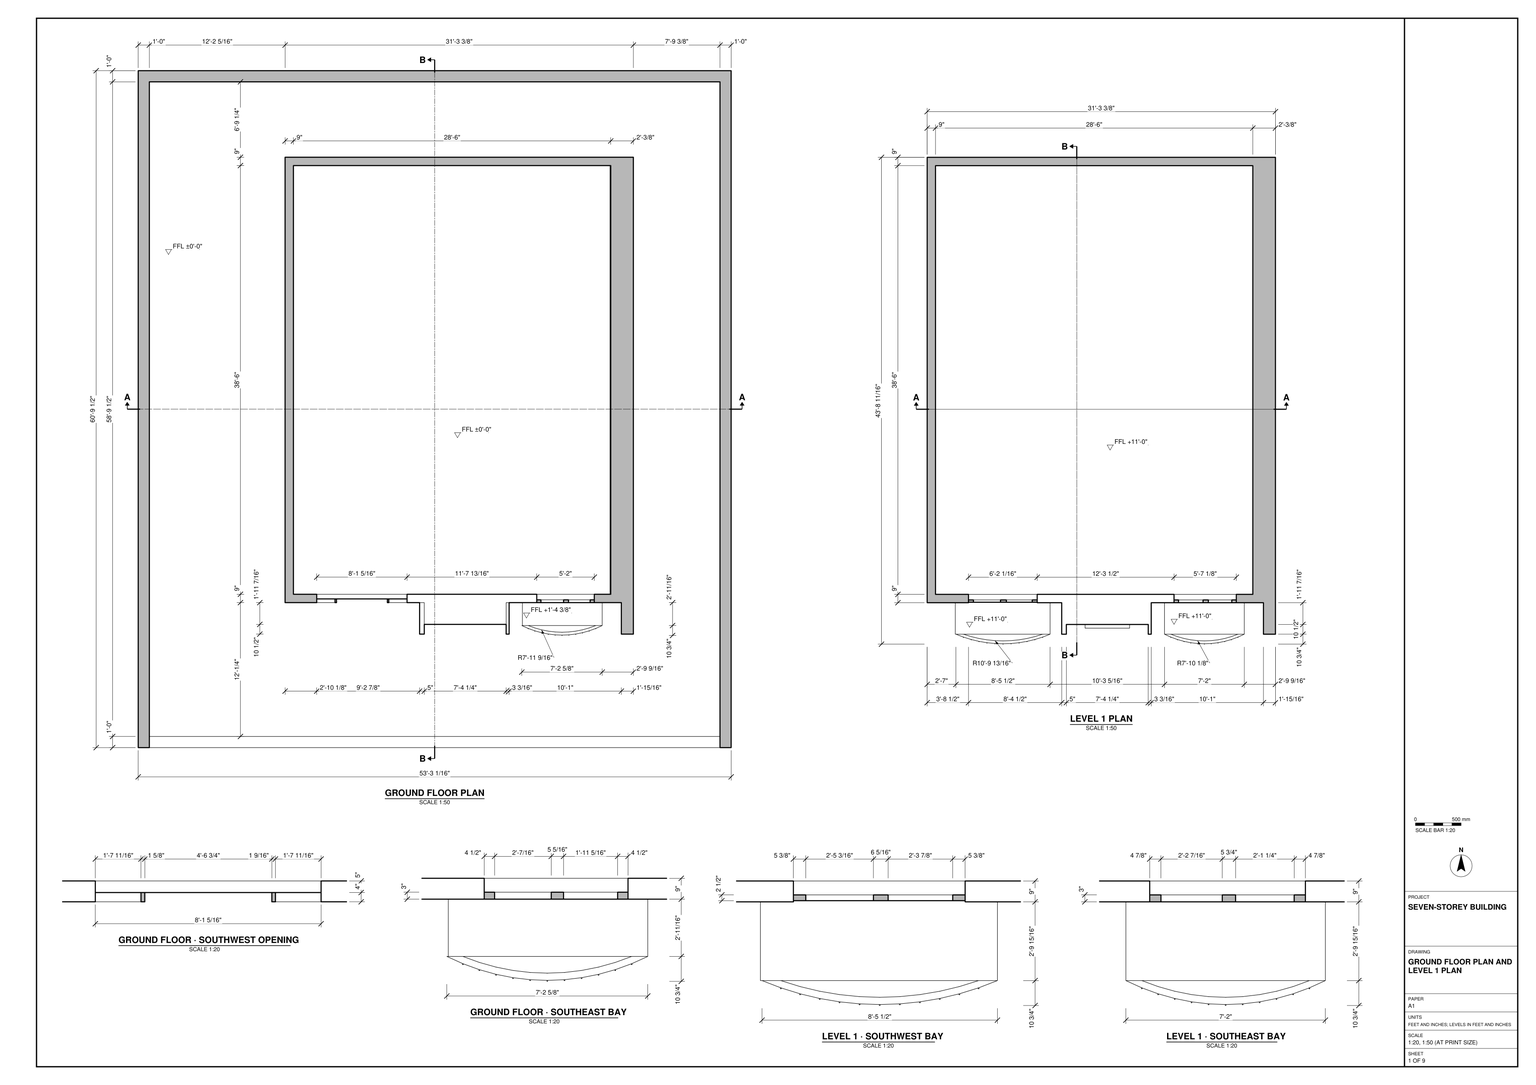
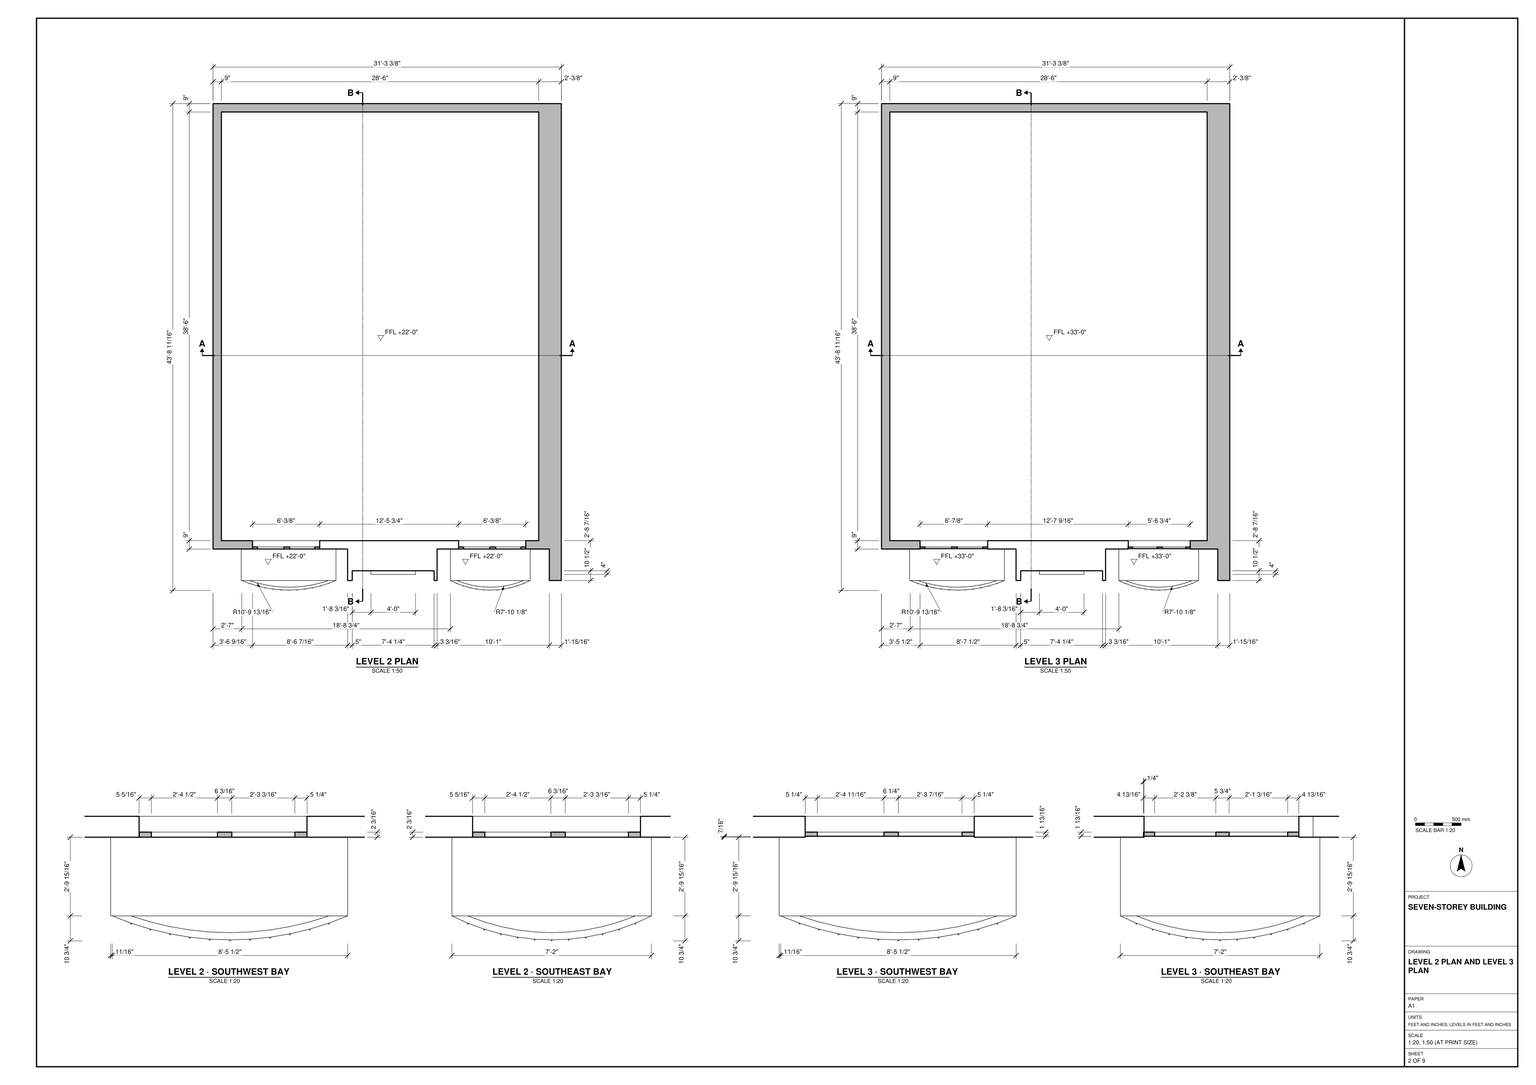
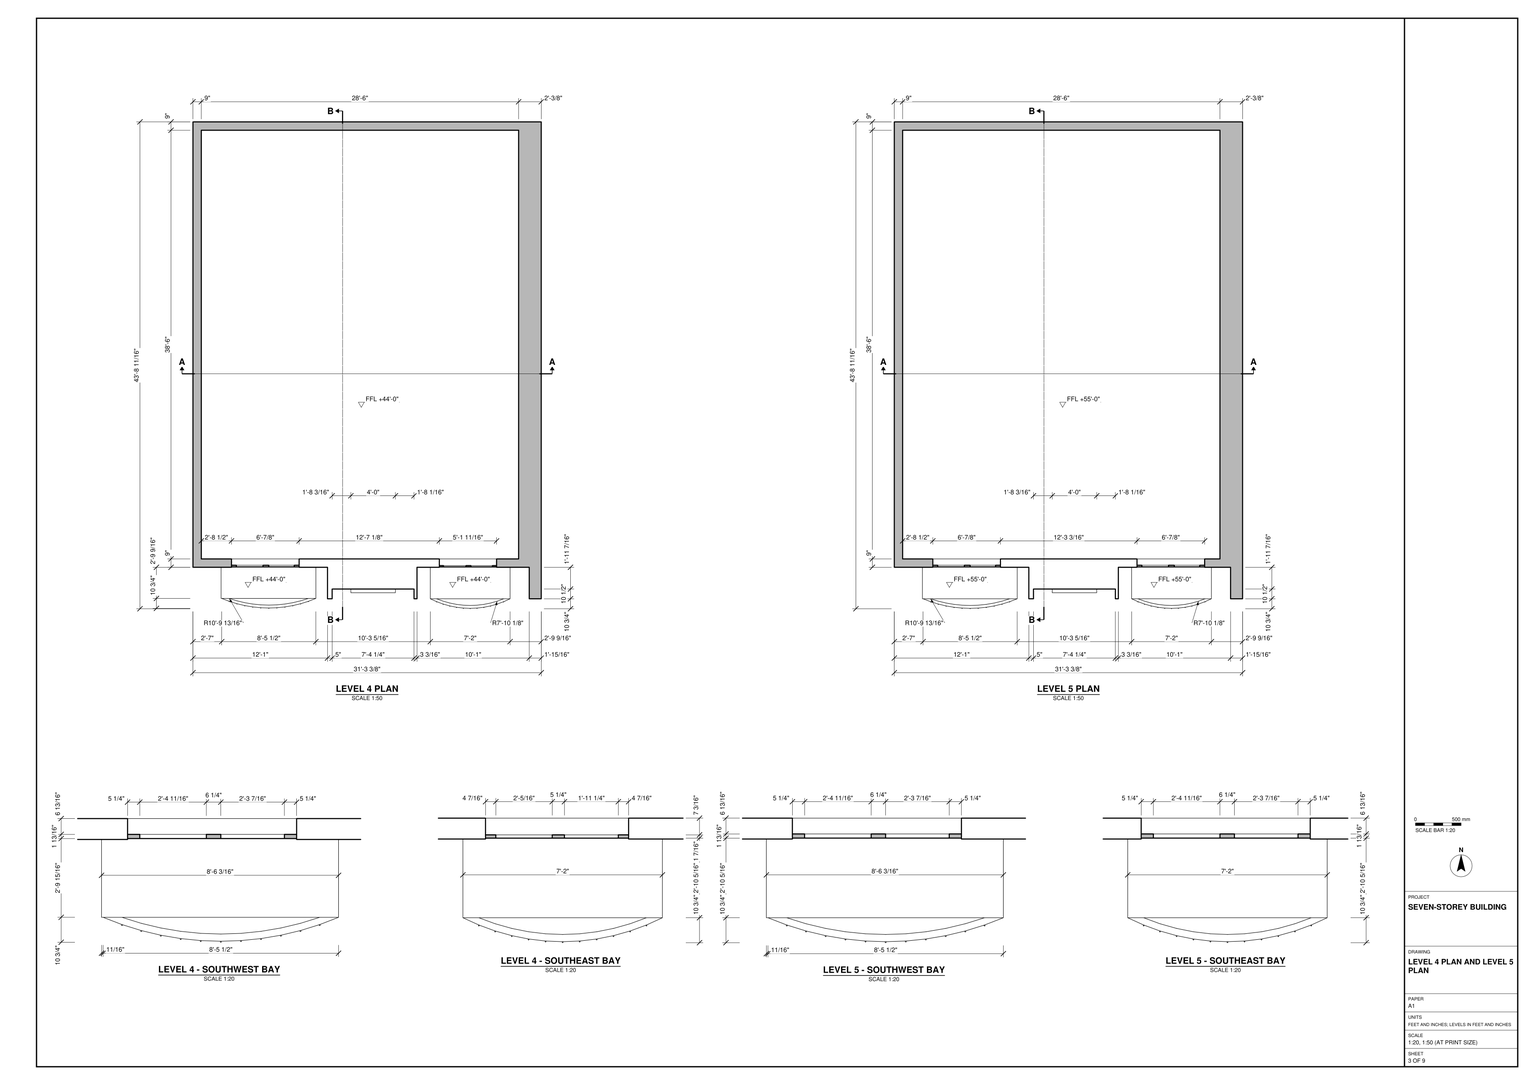
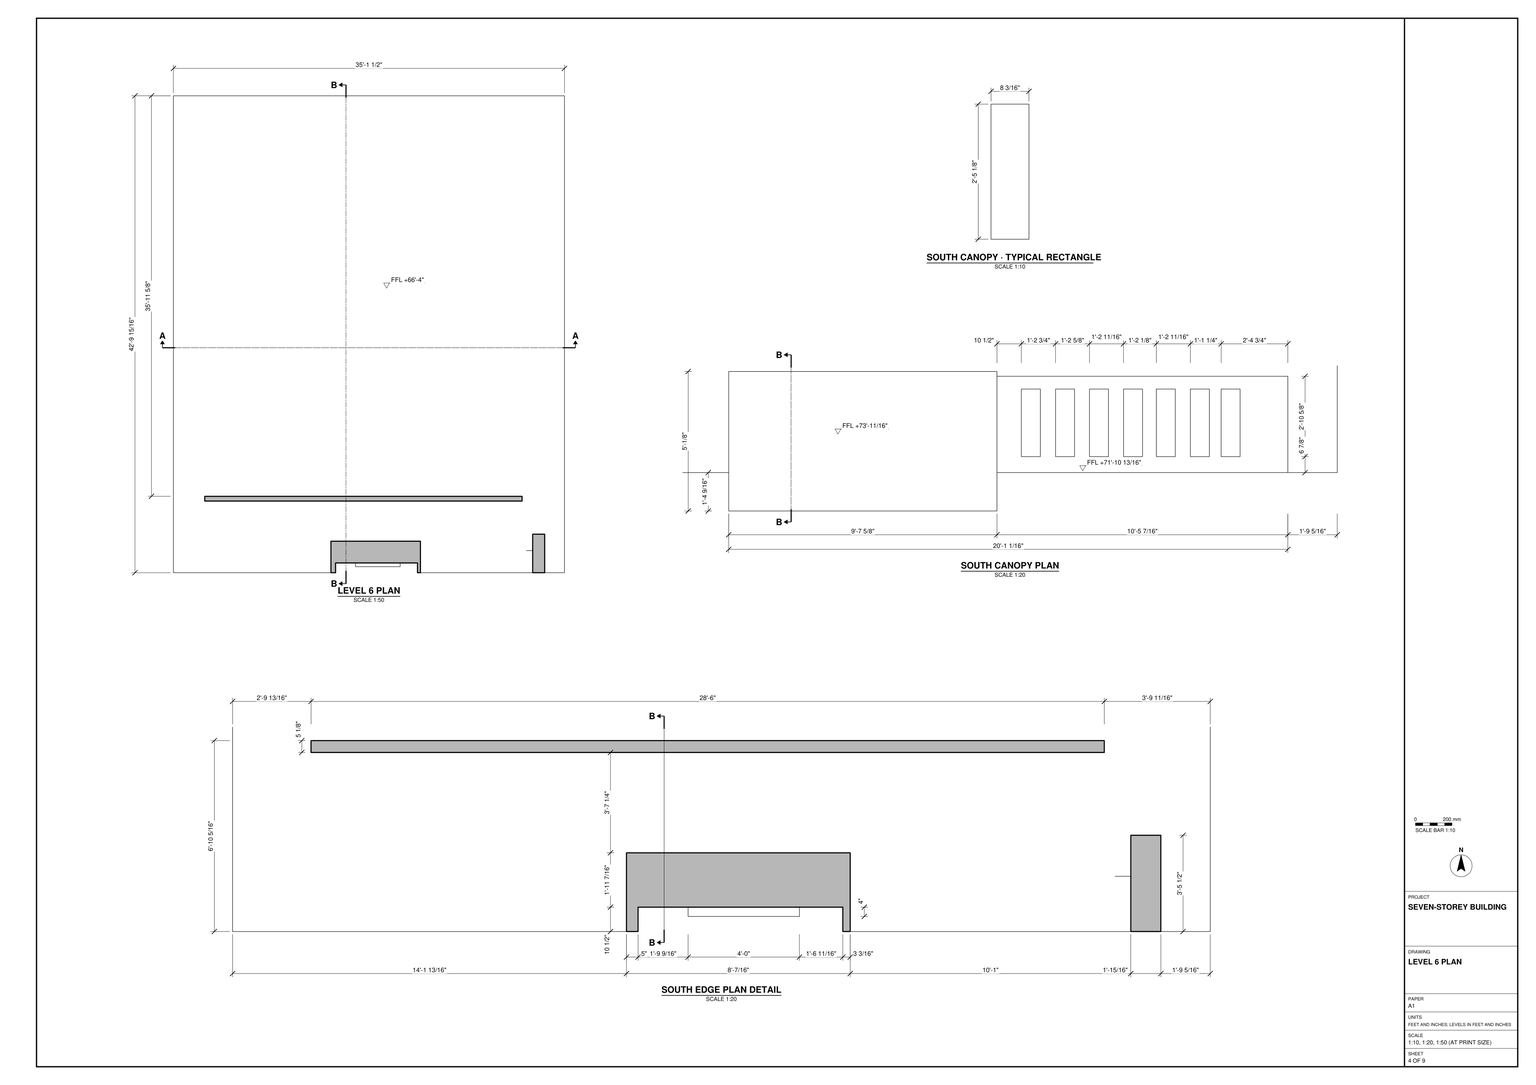
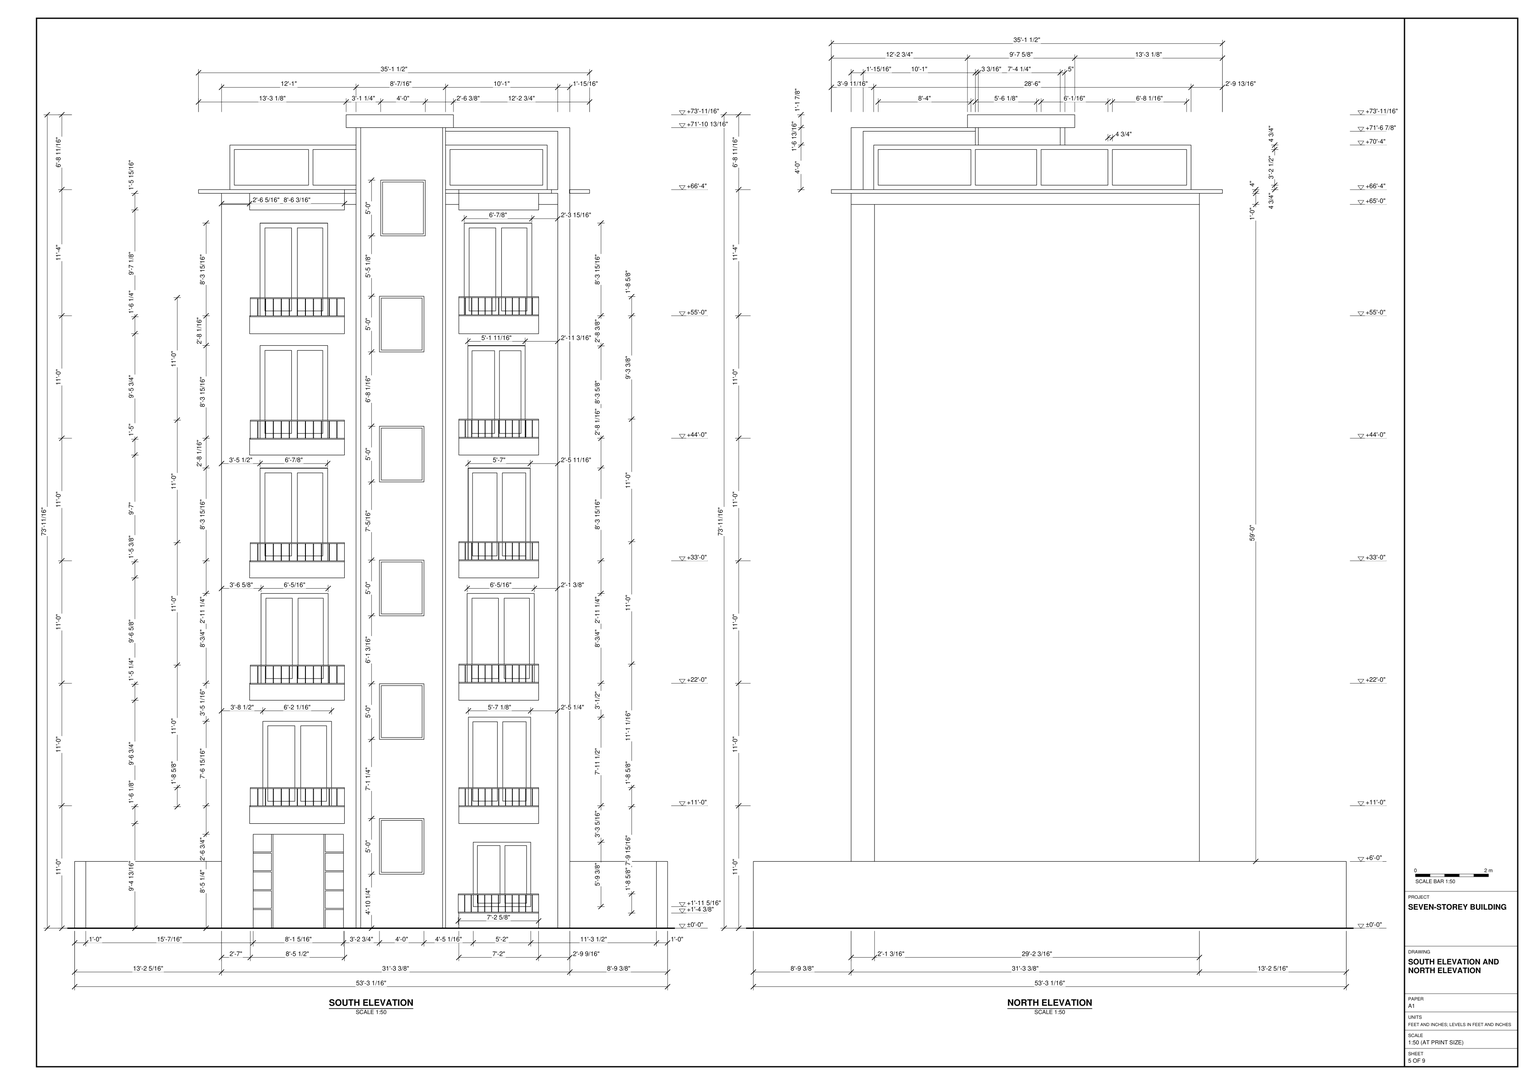
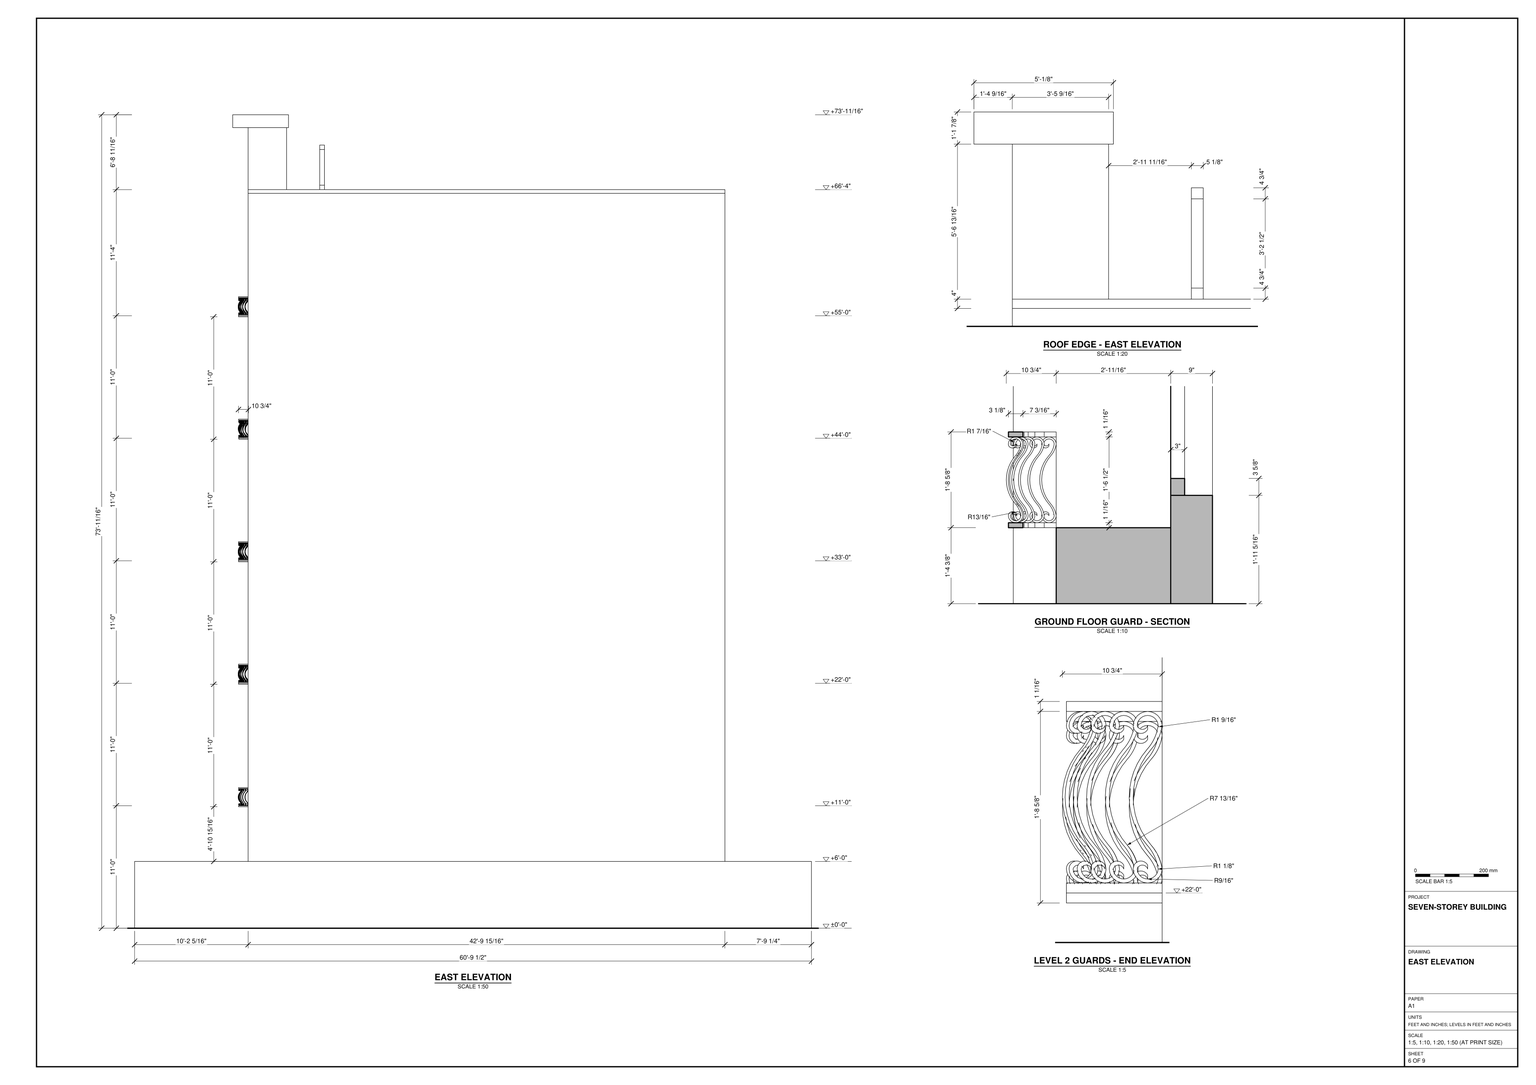
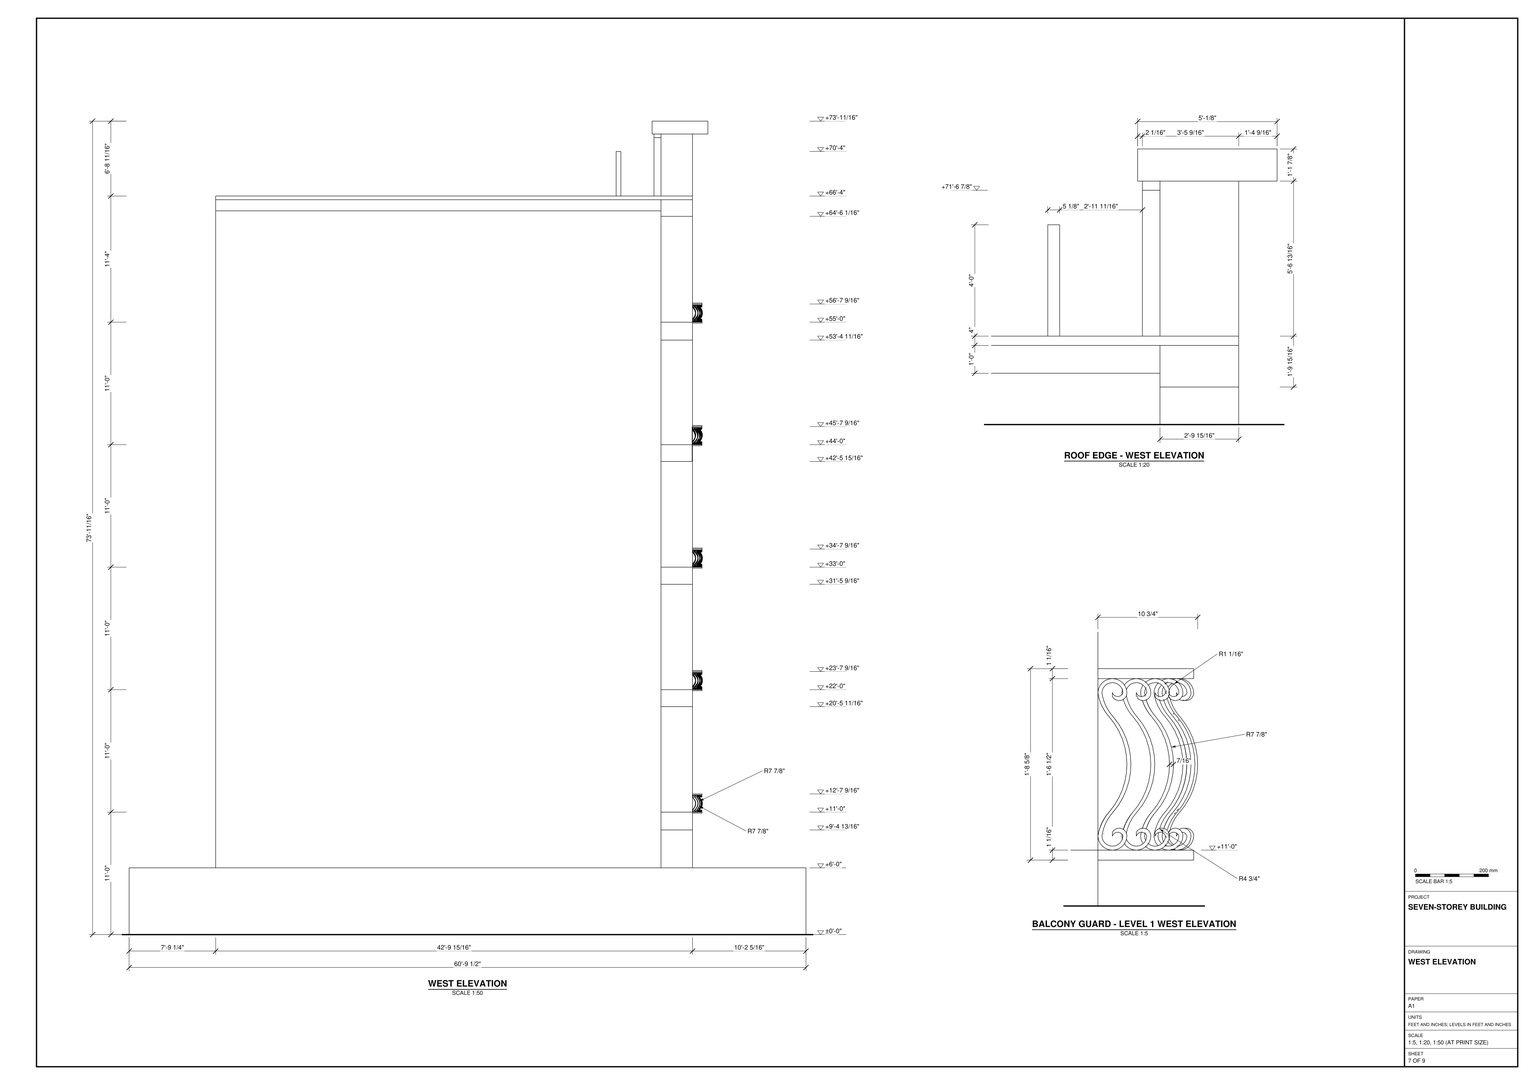
Build the seven-storey building and its site enclosure in SketchUp using task_files/diagram_01.pdf. Work in feet and inches. With the south façade facing the open end of the enclosure, the complete model should measure 53'-3 1/16" along X, 60'-9 1/2" along Y and 73'-11/16" along Z. Set the levels relative to the ground floor at ±0'-0", +11'-0", +22'-0", +33'-0", +44'-0", +55'-0" and +66'-4".

Use the ground floor plan to position the building inside the three-sided site enclosure. Follow the setbacks on each side rather than centring the footprint. Model the exterior walls at their drawn thicknesses, including the thicker east wall and its return at the south façade. Use the sections to set out the floor slabs and roof.

Distinguish the straight southwest opening on the ground floor from the projecting southeast bay. On levels 1 through 5, model the paired balcony bays on either side of the central projection. Follow each level's plan and enlarged details for the opening widths, frame divisions, balcony outlines and curved rails. Include stairs, built-in joinery and main furniture only where shown. Decor and loose items shown may be represented by any suitable library component.

Keep shell elements such as walls, slabs and roof, and each furniture or joinery piece, in separate groups or components. Use components for repeated parts such as matching balcony rails. Save one SketchUp model as output_files/seven_storey_building_with_curved_balcony_rails.skp.

# SketchUp Ruby script. Lengths in inches.
U = 1.inch
M = Sketchup.active_model
def pt(a) = Geom::Point3d.new(a.map { |v| v * U })
def face(e, loops, mat)
  f = e.add_face(loops[0].map { |a| pt(a) })
  loops[1..].each { |l| e.add_face(l.map { |a| pt(a) }).erase! }
  f.material = f.back_material = mat if mat
  f
end
# faces: each face lists its corners as indices into pts; further lists are holes
def faces(e, pts, list, mat = nil) = list.each { |f| face(e, (f[0].is_a?(Array) ? f : [f]).map { |l| l.map { |i| pts[i] } }, mat) }
# xy, xz, yz: faces in a plane at the given z, y or x. An outline is a flat list of corners, or four numbers for a rectangle; further outlines are holes
def ring(l) = l.size == 4 ? [[l[0], l[1]], [l[2], l[1]], [l[2], l[3]], [l[0], l[3]]] : l.each_slice(2).to_a
def flat(e, list, mat, &to3) = list.each { |f| face(e, (f[0].is_a?(Array) ? f : [f]).map { |l| ring(l).map { |u, v| to3.(u, v) } }, mat) }
def xy(e, z, list, mat = nil) = flat(e, list, mat) { |x, y| [x, y, z] }
def xz(e, y, list, mat = nil) = flat(e, list, mat) { |x, z| [x, y, z] }
def yz(e, x, list, mat = nil) = flat(e, list, mat) { |y, z| [x, y, z] }
def lines(e, pts, list) = list.each { |a, b| e.add_line(pt(pts[a]), pt(pts[b])) }
# prism: a flat outline (further loops are holes) pulled along v
def prism(e, loops, v, mat = nil)
  f = face(e, loops, mat); d = Geom::Vector3d.new(v.map { |x| x * U })
  f.pushpull(f.normal.samedirection?(d) ? d.length : -d.length)
end
def box(e, o, s, mat = nil) = prism(e, [[o, [o[0] + s[0], o[1], o[2]], [o[0] + s[0], o[1] + s[1], o[2]], [o[0], o[1] + s[1], o[2]]]], [0, 0, s[2]], mat)
def at(x, y, z, deg = 0) = Geom::Transformation.translation(pt([x, y, z])) * Geom::Transformation.rotation(ORIGIN, Z_AXIS, deg.degrees)
def axes(o, x, y, z) = Geom::Transformation.new([*x, 0, *y, 0, *z, 0, *pt(o).to_a, 1])
def part(name) = M.definitions.add(name)
# library, detail: a bought-in or finely detailed component or shape, given as its bounding box
def library(name, o, s) = part(name).tap { |d| box(d.entities, o, s) }
def detail(e, o, s) = box(e.add_group.entities, o, s)
def put(e, d, t, mat = nil) = e.add_instance(d, t).tap { |i| i.material = mat if mat }
def group(e, t, mat = nil) = e.add_group.tap { |g| g.transformation = t; g.material = mat if mat }.entities
root = M.entities
M.materials.add("[Blinds Wood Bamboo]").color = [131, 94, 60]
M.materials.add("[Stone Coursed Rough]").color = [165, 160, 130]
M.materials.add("[Stone Flagstone Ashlar]").color = [175, 116, 102]
M.materials.add("[Stone Sandstone Ashlar Light]").color = [206, 178, 128]
M.materials.add("[Translucent Glass Blue]").color = [100, 149, 237]
M.materials["[Translucent Glass Blue]"].alpha = 0.5
M.materials.add("[Translucent Glass Dark Green]").color = [62, 91, 5]
M.materials["[Translucent Glass Dark Green]"].alpha = 0.5
M.materials.add("[Wood Floor Parquet]").color = [145, 89, 39]
c1 = library("Balcony Rail",[43,-55.5,71],[118,12.5,24])
c2 = part("Group\#1")
xy(c2.entities,0,[[0,0,37.3125,6]])
xy(c2.entities,2.69,[[2.69,0,17.39,6],[20.58,0,34.62,6]])
xy(c2.entities,48.62,[[2.69,0,17.39,6],[20.58,0,34.62,6]])
xy(c2.entities,51.3125,[[0,0,37.3125,6]])
xz(c2.entities,0,[[[0,0,37.3125,51.3125],[2.69,2.69,17.39,48.62],[20.58,2.69,34.62,48.62]]])
xz(c2.entities,0,[[2.69,2.69,17.39,48.62],[20.58,2.69,34.62,48.62]],"[Translucent Glass Blue]")
xz(c2.entities,6,[[[0,0,37.3125,51.3125],[2.69,2.69,34.62,48.62]],[17.39,2.69,20.58,48.62]])
yz(c2.entities,0,[[0,0,6,51.3125]])
yz(c2.entities,2.69,[[0,2.69,6,48.62]])
yz(c2.entities,17.39,[[0,2.69,6,48.62]])
yz(c2.entities,20.58,[[0,2.69,6,48.62]])
yz(c2.entities,34.62,[[0,2.69,6,48.62]])
yz(c2.entities,37.3125,[[0,0,6,51.3125]])
xy(root,0,[[303.3,122.31,308.3,156.25],[396.57,122.31,399.76,156.25],[520.74,122.31,520.74,156.25,508.49,156.25,508.49,165.25,509.3,165.25,509.3,627.25,508.49,627.25,508.49,636.25,533.67,636.25,533.67,122.31],[414.08,131.56,500.08,156.25],[308.3,132.81,308.3,156.25,289.75,156.25,289.75,165.25,508.49,165.25,508.49,156.25,396.57,156.25,396.57,132.81],
  [158.3,156.25,158.3,636.25,508.49,636.25,508.49,627.25,167.3,627.25,167.3,165.25,192.42,165.25,192.42,156.25],[167.3,165.25,508.49,627.25],[508.49,165.25,509.3,627.25]])
xy(root,16.375,[[414.08,131.56,500.08,156.25]])
xy(root,23.34,[[429.57,156.25,491.57,165.25]])
xy(root,58.24,[[328.5,128.81,376.5,132.81]])
xy(root,60.24,[[330.5,128.81,374.5,132.81]])
xy(root,92.72,[[429.57,156.25,491.57,165.25]])
xy(root,101.23,[[192.42,156.25,289.75,165.25]])
xy(root,112.8125,[[188.6,122.31,290.78,156.25],[414.08,122.31,500.08,156.25]])
xy(root,114,[[167.3,165.25,509.3,627.25]])
xy(root,116.24,[[330.5,128.81,374.5,132.81]])
xy(root,118.24,[[328.5,128.81,376.5,132.81]])
xy(root,120,[[167.3,165.25,509.3,627.25]])
xy(root,132,[[188.6,122.31,290.78,122.31,290.78,156.25,276.87,156.25,276.87,165.25,202.83,165.25,202.83,156.25,188.6,156.25],[414.08,122.31,500.08,122.31,500.08,156.25,491.48,156.25,491.48,165.25,424.35,165.25,424.35,156.25,414.08,156.25],[167.3,165.25,509.3,627.25]])
xy(root,203.49,[[328.5,128.81,376.5,132.81]])
xy(root,205.49,[[330.5,128.81,374.5,132.81]])
xy(root,222.96,[[202.83,156.25,276.87,165.25]])
xy(root,227.51,[[424.35,156.25,491.48,165.25]])
xy(root,245.6875,[[188.6,122.31,290.78,156.25],[414.08,122.31,500.08,156.25]])
xy(root,246.5625,[[167.3,165.25,509.3,627.25]])
xy(root,260.5625,[[422.98,156.25,495.37,165.25]])
xy(root,261.49,[[330.5,128.81,374.5,132.81]])
xy(root,261.5625,[[200.86,156.25,273.24,165.25]])
xy(root,263.49,[[328.5,128.81,376.5,132.81]])
xy(root,264,[[188.6,122.31,290.78,122.31,290.78,156.25,273.24,156.25,273.24,165.25,200.86,165.25,200.86,156.25,188.6,156.25],[414.08,122.31,500.08,122.31,500.08,156.25,495.37,156.25,495.37,165.25,422.98,165.25,422.98,156.25,414.08,156.25],[167.3,165.25,509.3,627.25]])
xy(root,336.68,[[328.5,128.81,376.5,132.81]])
xy(root,338.68,[[330.5,128.81,374.5,132.81]])
xy(root,360.76,[[200.86,156.25,273.24,165.25],[422.98,156.25,495.37,165.25]])
xy(root,377.5625,[[188.6,122.31,290.78,156.25],[414.08,122.31,500.08,156.25]])
xy(root,378,[[167.3,165.25,509.3,627.25]])
xy(root,394.68,[[330.5,128.81,374.5,132.81]])
xy(root,396,[[188.6,122.31,290.78,122.31,290.78,156.25,272.71,156.25,272.71,165.25,199.83,165.25,199.83,156.25,188.6,156.25],[414.08,122.31,500.08,122.31,500.08,156.25,491.02,156.25,491.02,165.25,424.26,165.25,424.26,156.25,414.08,156.25],[491.02,156.25,497.15,165.25],[167.3,165.25,509.3,627.25]])
xy(root,396.68,[[328.5,128.81,376.5,132.81]])
xy(root,480.99,[[328.5,128.81,376.5,132.81]])
xy(root,482.99,[[330.5,128.81,374.5,132.81]])
xy(root,495.61,[[199.83,156.25,272.71,165.25],[424.26,156.25,491.02,165.25]])
xy(root,509.9375,[[414.08,122.31,500.08,156.25],[188.6,122.68,290.78,156.25]])
xy(root,510,[[167.3,165.25,509.3,627.25]])
xy(root,528,[[414.08,122.31,500.08,122.31,500.08,156.25,485.52,156.25,485.52,165.25,423.83,165.25,423.83,156.25,414.08,156.25],[188.6,122.68,290.78,122.68,290.78,156.25,272.71,156.25,272.71,165.25,199.83,165.25,199.83,156.25,188.6,156.25],[167.3,165.25,509.3,627.25]])
xy(root,538.99,[[330.5,128.81,374.5,132.81]])
xy(root,540.99,[[328.5,128.81,376.5,132.81]])
xy(root,621.05,[[328.5,128.81,376.5,132.81]])
xy(root,623.05,[[330.5,128.81,374.5,132.81]])
xy(root,627.99,[[199.83,156.25,272.71,165.25],[423.83,156.25,485.52,165.25]])
xy(root,640.6875,[[188.6,122.31,290.78,156.25],[414.08,122.31,500.08,156.25]])
xy(root,642,[[167.3,165.25,509.3,627.25]])
xy(root,660,[[188.6,122.31,290.78,122.31,290.78,156.25,272.71,156.25,272.71,165.25,199.83,165.25,199.83,156.25,188.6,156.25],[414.08,122.31,500.08,122.31,500.08,156.25,492.77,156.25,492.77,165.25,419.89,165.25,419.89,156.25,414.08,156.25],[167.3,165.25,509.3,627.25]])
xy(root,679.05,[[330.5,128.81,374.5,132.81]])
xy(root,681.05,[[328.5,128.81,376.5,132.81]])
xy(root,746.18,[[329.87,128.81,377.87,132.81]])
xy(root,748.18,[[331.87,128.81,375.87,132.81]])
xy(root,759.8,[[199.83,156.25,272.71,165.25],[419.89,156.25,492.77,165.25]])
xy(root,774.0625,[[188.6,122.31,290.78,156.25],[414.08,122.31,500.08,156.25]])
xy(root,780,[[158.3,156.25,158.3,636.25,508.49,636.25,508.49,627.25,167.3,627.25,167.3,156.25],[167.3,156.25,508.49,165.25],[508.49,156.25,509.3,165.25],[167.3,165.25,508.49,627.25],[508.49,165.25,509.3,627.25]])
xy(root,792,[[133.49,122.31,158.3,636.25],[158.3,122.31,167.3,156.25],[167.3,122.31,188.6,156.25],[188.6,122.31,290.78,156.25],[290.78,122.31,303.3,156.25],
  [399.76,122.31,414.08,156.25],[414.08,122.31,500.08,156.25],[500.08,122.31,500.08,156.25,513.92,156.25,513.92,146.12,520.74,146.12,520.74,122.31],[533.3,122.31,554.99,156.25],[513.92,146.12,520.74,156.25],
  [158.3,156.25,158.3,636.25,533.67,636.25,533.67,163.81,533.3,163.81,533.3,156.25,509.3,156.25,509.3,627.25,167.3,627.25,167.3,156.25],[167.3,156.25,509.3,165.25],[533.3,156.25,533.67,163.81],[533.67,156.25,554.99,636.25]])
xy(root,796,[[[133.49,122.31,303.3,122.31,303.3,156.25,399.76,156.25,399.76,122.31,520.74,122.31,520.74,163.81,533.3,163.81,533.3,122.31,554.99,122.31,554.99,636.25,133.49,636.25],[167.3,199.49,509.3,204.61]],[520.74,156.25,533.3,163.81]])
xy(root,804.18,[[331.87,128.81,375.87,132.81]])
xy(root,806.18,[[329.87,128.81,377.87,132.81]])
xy(root,844,[[167.3,199.49,509.3,204.61]])
xy(root,858.875,[[[399.76,122.31,520.74,163.81],[418.78,129.18,426.97,158.31],[433.53,129.18,441.72,158.31],[448.15,129.18,456.34,158.31],[462.84,129.18,471.03,158.31],[476.97,129.18,485.15,158.31],[491.65,129.18,499.84,158.31],[504.9,129.18,513.09,158.31]]])
xy(root,862.8125,[[292.61,105.75,303.3,165.87],[303.3,105.75,308.3,122.31],[308.3,105.75,396.57,132.81],[396.57,105.75,399.76,122.31],[399.76,105.75,408.26,122.31],
  [303.3,122.31,303.3,156.25,399.76,156.25,399.76,132.81,308.3,132.81,308.3,122.31],[396.57,122.31,399.76,132.81],[399.76,122.31,408.26,132.81],[[408.26,122.31,533.67,163.81],[418.78,129.18,426.97,158.31],[433.53,129.18,441.72,158.31],[448.15,129.18,456.34,158.31],[462.84,129.18,471.03,158.31],[476.97,129.18,485.15,158.31],[491.65,129.18,499.84,158.31],[504.9,129.18,513.09,158.31]],[399.76,132.81,408.26,163.81],
  [303.3,156.25,308.3,165.87],[308.3,156.25,396.57,165.87],[396.57,156.25,399.76,165.87],[399.76,163.81,408.26,165.87]])
xy(root,876.6875,[[292.61,105.75,408.26,165.87]])
xz(root,105.75,[[292.61,862.8125,408.26,876.6875]])
xz(root,122.31,[[520.74,0,533.67,0,533.67,792,533.3,792,533.3,796,533.67,796,533.67,862.8125,399.76,862.8125,399.76,858.875,520.74,858.875,520.74,796,513.92,796,513.92,792,520.74,792],[188.6,112.8125,290.78,132],[414.08,112.8125,500.08,132],[188.6,245.6875,290.78,264],[414.08,245.6875,500.08,264],
  [188.6,377.5625,290.78,396],[414.08,377.5625,500.08,396],[414.08,509.9375,500.08,528],[188.6,640.6875,290.78,660],[414.08,640.6875,500.08,660],
  [188.6,774.0625,290.78,792],[414.08,774.0625,500.08,792],[133.49,792,290.78,796],[290.78,792,303.3,796],[399.76,792,414.08,796],
  [414.08,792,513.92,796],[533.3,792,533.67,796],[533.67,792,554.99,796]])
xz(root,122.31,[[303.3,0,308.3,862.8125],[396.57,0,399.76,862.8125]],"[Stone Flagstone Ashlar]")
xz(root,122.68,[[188.6,509.9375,290.78,528]])
xz(root,128.81,[[[328.5,58.24,376.5,118.24],[330.5,60.24,374.5,116.24]],[[328.5,203.49,376.5,263.49],[330.5,205.49,374.5,261.49]],[[328.5,336.68,376.5,396.68],[330.5,338.68,374.5,394.68]],[[328.5,480.99,376.5,540.99],[330.5,482.99,374.5,538.99]],[[328.5,621.05,376.5,681.05],[330.5,623.05,374.5,679.05]],
  [[329.87,746.18,377.87,806.18],[331.87,748.18,375.87,804.18]]])
xz(root,129.18,[[418.78,858.875,426.97,862.8125],[433.53,858.875,441.72,862.8125],[448.15,858.875,456.34,862.8125],[462.84,858.875,471.03,862.8125],[476.97,858.875,485.15,862.8125],
  [491.65,858.875,499.84,862.8125],[504.9,858.875,513.09,862.8125]])
xz(root,131.56,[[414.08,0,500.08,16.375]])
xz(root,132.81,[[[328.5,621.05,376.5,681.05],[330.5,623.05,374.5,679.05]],[[329.87,746.18,377.87,806.18],[331.87,748.18,375.87,804.18]]])
xz(root,132.81,[[[308.3,0,396.57,862.8125],[328.5,58.24,376.5,118.24],[328.5,203.49,376.5,263.49],[328.5,336.68,376.5,396.68],[328.5,480.99,376.5,540.99],[328.5,621.05,376.5,681.05],[329.87,746.18,377.87,806.18]]],"[Stone Coursed Rough]")
xz(root,132.81,[[330.5,60.24,374.5,116.24],[330.5,205.49,374.5,261.49],[330.5,338.68,374.5,394.68],[330.5,482.99,374.5,538.99],[330.5,623.05,374.5,679.05],
  [331.87,748.18,375.87,804.18]],"[Translucent Glass Blue]")
xz(root,156.25,[[[158.3,0,192.42,0,192.42,101.23,289.75,101.23,289.75,0,303.3,0,303.3,780,290.78,780,290.78,774.0625,188.6,774.0625,188.6,780,158.3,780],[188.6,640.6875,188.6,660,199.83,660,199.83,759.8,272.71,759.8,272.71,660,290.78,660,290.78,640.6875],[188.6,377.5625,188.6,396,199.83,396,199.83,495.61,272.71,495.61,272.71,396,290.78,396,290.78,377.5625],[188.6,509.9375,188.6,528,199.83,528,199.83,627.99,272.71,627.99,272.71,528,290.78,528,290.78,509.9375],[188.6,245.6875,188.6,264,200.86,264,200.86,360.76,273.24,360.76,273.24,264,290.78,264,290.78,245.6875],[188.6,112.8125,188.6,132,202.83,132,202.83,222.96,276.87,222.96,276.87,132,290.78,132,290.78,112.8125]],[[399.76,0,414.08,0,414.08,16.375,500.08,16.375,500.08,0,520.74,0,520.74,780,500.08,780,500.08,774.0625,414.08,774.0625,414.08,780,399.76,780],[414.08,640.6875,414.08,660,419.89,660,419.89,759.8,492.77,759.8,492.77,660,500.08,660,500.08,640.6875],[414.08,245.6875,414.08,264,422.98,264,422.98,360.76,495.37,360.76,495.37,264,500.08,264,500.08,245.6875],[414.08,377.5625,414.08,396,424.26,396,424.26,495.61,491.02,495.61,491.02,396,500.08,396,500.08,377.5625],[414.08,112.8125,414.08,132,424.35,132,424.35,227.51,491.48,227.51,491.48,132,500.08,132,500.08,112.8125],[414.08,509.9375,414.08,528,423.83,528,423.83,627.99,485.52,627.99,485.52,528,500.08,528,500.08,509.9375],[429.57,23.34,491.57,92.72]],[414.08,0,500.08,16.375],[188.6,112.8125,290.78,120],[414.08,112.8125,500.08,120],
  [188.6,245.6875,290.78,252],[414.08,245.6875,500.08,252],[188.6,252,188.6,264,200.86,264,200.86,261.5625,273.24,261.5625,273.24,264,290.78,264,290.78,252],[414.08,252,414.08,264,422.98,264,422.98,260.5625,495.37,260.5625,495.37,264,500.08,264,500.08,252],[188.6,377.5625,290.78,384],
  [414.08,377.5625,500.08,384],[188.6,509.9375,290.78,516],[414.08,509.9375,500.08,516],[188.6,640.6875,290.78,648],[414.08,640.6875,500.08,648],
  [188.6,774.0625,290.78,780],[414.08,774.0625,500.08,780],[158.3,780,188.6,792],[188.6,780,290.78,792],[290.78,780,303.3,792],
  [303.3,780,308.3,792],[308.3,780,396.57,792],[396.57,780,399.76,792],[399.76,780,414.08,792],[414.08,780,500.08,792],
  [500.08,780,520.74,792],[303.3,792,308.3,796],[308.3,792,396.57,796],[396.57,792,399.76,796],[303.3,796,308.3,862.8125],
  [308.3,796,396.57,862.8125],[396.57,796,399.76,862.8125]])
xz(root,158.31,[[418.78,858.875,426.97,862.8125],[433.53,858.875,441.72,862.8125],[448.15,858.875,456.34,862.8125],[462.84,858.875,471.03,862.8125],[476.97,858.875,485.15,862.8125],
  [491.65,858.875,499.84,862.8125],[504.9,858.875,513.09,862.8125]])
xz(root,163.81,[[533.3,792,533.3,796,520.74,796,520.74,858.875,399.76,858.875,399.76,862.8125,533.67,862.8125,533.67,792]])
xz(root,165.25,[[[167.3,0,167.3,114,509.3,114,509.3,0,289.75,0,289.75,101.23,192.42,101.23,192.42,0],[429.57,23.34,491.57,92.72]],[167.3,114,509.3,120],[167.3,120,509.3,132],[167.3,132,167.3,246.5625,509.3,246.5625,509.3,132,491.48,132,491.48,227.51,424.35,227.51,424.35,132,276.87,132,276.87,222.96,202.83,222.96,202.83,132],[167.3,246.5625,509.3,252],
  [167.3,252,167.3,264,200.86,264,200.86,261.5625,273.24,261.5625,273.24,264,422.98,264,422.98,260.5625,495.37,260.5625,495.37,264,509.3,264,509.3,252],[422.98,260.5625,495.37,264],[200.86,261.5625,273.24,264],[167.3,264,167.3,378,509.3,378,509.3,264,495.37,264,495.37,360.76,422.98,360.76,422.98,264,273.24,264,273.24,360.76,200.86,360.76,200.86,264],[167.3,378,509.3,384],
  [167.3,384,509.3,396],[167.3,396,167.3,510,509.3,510,509.3,396,497.15,396,497.15,495.61,424.26,495.61,424.26,396,272.71,396,272.71,495.61,199.83,495.61,199.83,396],[491.02,396,497.15,495.61],[167.3,510,509.3,528],[167.3,528,167.3,642,509.3,642,509.3,528,485.52,528,485.52,627.99,423.83,627.99,423.83,528,272.71,528,272.71,627.99,199.83,627.99,199.83,528],
  [167.3,660,167.3,780,509.3,780,509.3,660,492.77,660,492.77,759.8,419.89,759.8,419.89,660,272.71,660,272.71,759.8,199.83,759.8,199.83,660],[167.3,780,509.3,792]])
xz(root,165.87,[[292.61,862.8125,408.26,876.6875]])
xz(root,199.49,[[[167.3,796,509.3,844],[404.5625,800.76,504.53,839.24],[172.0625,800.76,252.12,839.24],[256.875,800.76,328.93,839.24],[333.6875,800.76,399.81,839.24]]])
xz(root,199.49,[[172.0625,800.76,252.12,839.24],[256.875,800.76,328.93,839.24],[333.6875,800.76,399.81,839.24],[404.5625,800.76,504.53,839.24]],"[Translucent Glass Blue]")
xz(root,204.61,[[[167.3,796,509.3,844],[404.5625,800.76,504.53,839.24],[172.0625,800.76,252.12,839.24],[256.875,800.76,328.93,839.24],[333.6875,800.76,399.81,839.24]]])
xz(root,204.61,[[172.0625,800.76,252.12,839.24],[256.875,800.76,328.93,839.24],[333.6875,800.76,399.81,839.24],[404.5625,800.76,504.53,839.24]],"[Translucent Glass Blue]")
xz(root,627.25,[[167.3,0,509.3,114],[167.3,114,509.3,120],[167.3,120,509.3,132],[167.3,132,509.3,246.5625],[167.3,246.5625,509.3,252],
  [167.3,252,509.3,264],[167.3,264,509.3,378],[167.3,378,509.3,384],[167.3,384,509.3,396],[167.3,396,509.3,510],
  [167.3,510,509.3,516],[167.3,516,509.3,528],[167.3,528,509.3,642],[167.3,642,509.3,648],[167.3,648,509.3,660],
  [167.3,660,509.3,780],[167.3,780,509.3,792]])
xz(root,636.25,[[158.3,0,508.49,780],[508.49,0,533.67,780],[158.3,780,533.67,792],[133.49,792,554.99,796]])
yz(root,133.49,[[122.31,792,636.25,796]])
yz(root,158.3,[[156.25,0,636.25,780],[156.25,780,636.25,792]])
yz(root,167.3,[[165.25,0,627.25,114],[165.25,114,182.37,120],[182.37,114,627.25,120],[165.25,120,182.37,132],[182.37,120,627.25,132],
  [165.25,132,627.25,246.5625],[165.25,246.5625,184.06,252],[184.06,246.5625,627.25,252],[165.25,252,184.06,264],[184.06,252,627.25,264],
  [165.25,264,627.25,378],[165.25,378,170.05,384],[170.05,378,180.74,384],[180.74,378,627.25,384],[165.25,384,170.05,396],
  [170.05,384,180.74,396],[180.74,384,627.25,396],[165.25,396,627.25,510],[165.25,510,196.48,516],[196.48,510,212.1,516],
  [212.1,510,627.25,516],[165.25,516,196.48,528],[196.48,516,212.1,528],[212.1,516,627.25,528],[165.25,528,627.25,642],
  [165.25,642,242.28,648],[242.28,642,263.78,648],[263.78,642,627.25,648],[165.25,648,242.28,660],[242.28,648,263.78,660],
  [263.78,648,627.25,660],[165.25,660,627.25,780],[165.25,780,627.25,792],[199.49,796,204.61,844]])
yz(root,188.6,[[122.31,112.8125,156.25,132],[122.31,245.6875,156.25,264],[122.31,377.5625,156.25,396],[122.68,509.9375,156.25,528],[122.31,640.6875,156.25,660],
  [122.31,774.0625,156.25,792]])
yz(root,192.42,[[156.25,0,165.25,101.23]])
yz(root,199.83,[[156.25,396,165.25,495.61],[156.25,528,165.25,627.99],[156.25,660,165.25,759.8]])
yz(root,200.86,[[156.25,261.5625,165.25,264],[156.25,264,165.25,360.76]])
yz(root,202.83,[[156.25,132,165.25,222.96]])
yz(root,272.71,[[156.25,396,165.25,495.61],[156.25,528,165.25,627.99],[156.25,660,165.25,759.8]])
yz(root,273.24,[[156.25,261.5625,165.25,264],[156.25,264,165.25,360.76]])
yz(root,276.87,[[156.25,132,165.25,222.96]])
yz(root,289.75,[[156.25,0,165.25,101.23]])
yz(root,290.78,[[122.31,112.8125,156.25,132],[122.31,245.6875,156.25,264],[122.31,377.5625,156.25,396],[122.68,509.9375,156.25,528],[122.31,640.6875,156.25,660],
  [122.31,774.0625,156.25,792]])
yz(root,292.61,[[105.75,862.8125,165.87,876.6875]])
yz(root,303.3,[[122.31,792,156.25,796],[122.31,796,156.25,862.8125]])
yz(root,303.3,[[122.31,0,156.25,792]],"[Stone Flagstone Ashlar]")
yz(root,308.3,[[122.31,792,132.81,796],[122.31,796,132.81,862.8125]])
yz(root,308.3,[[122.31,0,132.81,792]],"[Stone Flagstone Ashlar]")
yz(root,328.5,[[128.81,58.24,132.81,118.24],[128.81,203.49,132.81,263.49],[128.81,336.68,132.81,396.68],[128.81,480.99,132.81,540.99],[128.81,621.05,132.81,681.05]])
yz(root,329.87,[[128.81,746.18,132.81,806.18]])
yz(root,330.5,[[128.81,60.24,132.81,116.24],[128.81,205.49,132.81,261.49],[128.81,338.68,132.81,394.68],[128.81,482.99,132.81,538.99],[128.81,623.05,132.81,679.05]])
yz(root,331.87,[[128.81,748.18,132.81,804.18]])
yz(root,374.5,[[128.81,60.24,132.81,116.24],[128.81,205.49,132.81,261.49],[128.81,338.68,132.81,394.68],[128.81,482.99,132.81,538.99],[128.81,623.05,132.81,679.05]])
yz(root,375.87,[[128.81,748.18,132.81,804.18]])
yz(root,376.5,[[128.81,58.24,132.81,118.24],[128.81,203.49,132.81,263.49],[128.81,336.68,132.81,396.68],[128.81,480.99,132.81,540.99],[128.81,621.05,132.81,681.05]])
yz(root,377.87,[[128.81,746.18,132.81,806.18]])
yz(root,396.57,[[122.31,0,132.81,862.8125]],"[Stone Flagstone Ashlar]")
yz(root,399.76,[[122.31,792,156.25,796],[122.31,796,156.25,858.875],[122.31,858.875,156.25,862.8125],[156.25,858.875,163.81,862.8125]])
yz(root,399.76,[[122.31,0,156.25,792]],"[Stone Flagstone Ashlar]")
yz(root,408.26,[[105.75,862.8125,165.87,876.6875]])
yz(root,414.08,[[131.56,0,156.25,16.375],[122.31,112.8125,156.25,132],[122.31,245.6875,156.25,264],[122.31,377.5625,156.25,396],[122.31,509.9375,156.25,528],
  [122.31,640.6875,156.25,660],[122.31,774.0625,156.25,792]])
yz(root,418.78,[[129.18,858.875,158.31,862.8125]])
yz(root,419.89,[[156.25,660,165.25,759.8]])
yz(root,422.98,[[156.25,260.5625,165.25,264],[156.25,264,165.25,360.76]])
yz(root,423.83,[[156.25,528,165.25,627.99]])
yz(root,424.26,[[156.25,396,165.25,495.61]])
yz(root,424.35,[[156.25,132,165.25,227.51]])
yz(root,426.97,[[129.18,858.875,158.31,862.8125]])
yz(root,429.57,[[156.25,23.34,165.25,92.72]])
yz(root,433.53,[[129.18,858.875,158.31,862.8125]])
yz(root,441.72,[[129.18,858.875,158.31,862.8125]])
yz(root,448.15,[[129.18,858.875,158.31,862.8125]])
yz(root,456.34,[[129.18,858.875,158.31,862.8125]])
yz(root,462.84,[[129.18,858.875,158.31,862.8125]])
yz(root,471.03,[[129.18,858.875,158.31,862.8125]])
yz(root,476.97,[[129.18,858.875,158.31,862.8125]])
yz(root,485.15,[[129.18,858.875,158.31,862.8125]])
yz(root,485.52,[[156.25,528,165.25,627.99]])
yz(root,491.02,[[156.25,396,165.25,495.61]])
yz(root,491.48,[[156.25,132,165.25,227.51]])
yz(root,491.57,[[156.25,23.34,165.25,92.72]])
yz(root,491.65,[[129.18,858.875,158.31,862.8125]])
yz(root,492.77,[[156.25,660,165.25,759.8]])
yz(root,495.37,[[156.25,260.5625,165.25,264],[156.25,264,165.25,360.76]])
yz(root,499.84,[[129.18,858.875,158.31,862.8125]])
yz(root,500.08,[[131.56,0,156.25,16.375],[122.31,112.8125,156.25,132],[122.31,245.6875,156.25,264],[122.31,377.5625,156.25,396],[122.31,509.9375,156.25,528],
  [122.31,640.6875,156.25,660],[122.31,774.0625,156.25,792]])
yz(root,504.9,[[129.18,858.875,158.31,862.8125]])
yz(root,509.3,[[165.25,0,627.25,114],[165.25,114,627.25,120],[165.25,120,627.25,132],[165.25,132,627.25,246.5625],[165.25,246.5625,627.25,264],
  [165.25,264,627.25,378],[165.25,378,627.25,396],[165.25,396,627.25,510],[165.25,510,627.25,516],[165.25,516,627.25,528],
  [165.25,528,627.25,642],[165.25,642,627.25,648],[165.25,648,627.25,660],[165.25,660,627.25,780],[165.25,780,627.25,792],
  [199.49,796,204.61,800.76],[199.49,800.76,204.61,839.24],[199.49,839.24,204.61,844]])
yz(root,513.09,[[129.18,858.875,158.31,862.8125]])
yz(root,520.74,[[122.31,0,156.25,792],[122.31,796,163.81,858.875]])
yz(root,533.3,[[122.31,792,156.25,796],[156.25,792,163.81,796]])
yz(root,533.67,[[122.31,0,636.25,0,636.25,792,163.81,792,163.81,862.8125,122.31,862.8125]])
yz(root,554.99,[[122.31,792,636.25,796]])
# 12 loose lines left out
put(root,c1,axes([152.32,159.29,69.86],[0.86,0,0],[0,0.86,0],[0,0,0.86]))
put(root,c1,axes([152.32,159.29,201.86],[0.86,0,0],[0,0.86,0],[0,0,0.86]))
put(root,c1,axes([382.75,159.29,202.94],[0.72881,0,0],[0,0.86,0],[0,0,0.86]))
put(root,c1,axes([382.75,159.29,69.86],[0.72881,0,0],[0,0.86,0],[0,0,0.86]))
put(root,c1,axes([382.75,159.29,598.94],[0.72881,0,0],[0,0.86,0],[0,0,0.86]))
put(root,c1,axes([152.32,159.29,333.86],[0.86,0,0],[0,0.86,0],[0,0,0.86]))
put(root,c1,axes([382.75,159.29,466.94],[0.72881,0,0],[0,0.86,0],[0,0,0.86]))
put(root,c1,axes([152.32,159.29,597.86],[0.86,0,0],[0,0.86,0],[0,0,0.86]))
put(root,c1,axes([382.75,159.29,334.94],[0.72881,0,0],[0,0.86,0],[0,0,0.86]))
put(root,c1,axes([152.32,159.66,465.86],[0.86,0,0],[0,0.86,0],[0,0,0.86]))
put(root,c1,axes([381.88,168.54,-44.68],[0.73421,0,0],[0,0.86,0],[0,0,0.86]))
g1 = group(root,at(0,0,0))
xy(g1,0,[[12,0,627.0625,12],[12,12,627.0625,717.5]])
xy(g1,72,[[0,0,12,0,12,717.5,627.0625,717.5,627.0625,0,639.0625,0,639.0625,729.5,0,729.5]],"[Stone Sandstone Ashlar Light]")
xz(g1,0,[[0,0,12,72],[627.0625,0,639.0625,72]],"[Stone Sandstone Ashlar Light]")
xz(g1,717.5,[[12,0,627.0625,72]],"[Stone Sandstone Ashlar Light]")
xz(g1,729.5,[[0,0,639.0625,72]],"[Stone Sandstone Ashlar Light]")
yz(g1,0,[[0,0,729.5,72]],"[Stone Sandstone Ashlar Light]")
yz(g1,12,[[0,0,12,72],[12,0,717.5,72]],"[Stone Sandstone Ashlar Light]")
yz(g1,627.0625,[[0,0,12,72],[12,0,717.5,72]],"[Stone Sandstone Ashlar Light]")
yz(g1,639.0625,[[0,0,729.5,72]],"[Stone Sandstone Ashlar Light]")
put(root,c2,axes([423.05,156.25,264],[1.9383,0,0],[0,0.3652,0],[0,0,1.88562]))
put(root,c2,axes([423.83,156.625,528],[1.65353,0,0],[0,0.23658,0],[0,0,1.94142]))
put(root,c2,axes([429.57,156.25,23.34],[1.66164,0,0],[0,0.5,0],[0,0,1.35201]))
put(root,c2,axes([424.35,156.25,132],[1.79899,0,0],[0,0.5,0],[0,0,1.86136]))
put(root,c2,axes([202.83,156.76,132],[1.98433,0,0],[0,0.415,0],[0,0,1.77271]))
put(root,c2,axes([199.83,156.64,660],[1.95336,0,0],[0,0.29946,0],[0,0,1.94823]))
put(root,c2,axes([419.89,156.64,660],[1.95336,0,0],[0,0.29946,0],[0,0,1.94823]))
put(root,c2,axes([200.92,156.25,264],[1.9383,0,0],[0,0.3652,0],[0,0,1.88562]))
g2 = group(root,at(192.42,156.25,0))
xy(g2,0,[[19.69,0,21.33,4],[76.11,0,77.66,4]],"[Wood Floor Parquet]")
xy(g2,20.1,[[0,0,19.69,4],[77.66,0,97.33,4]],"[Wood Floor Parquet]")
xy(g2,21.46,[[0,0,19.69,4],[77.66,0,97.33,4]],"[Wood Floor Parquet]")
xy(g2,40.26,[[0,0,19.69,4],[77.66,0,97.33,4]],"[Wood Floor Parquet]")
xy(g2,41.62,[[0,0,19.69,4],[77.66,0,97.33,4]],"[Wood Floor Parquet]")
xy(g2,60.7,[[0,0,19.69,4],[77.66,0,97.33,4]],"[Wood Floor Parquet]")
xy(g2,62.06,[[0,0,19.69,4],[77.66,0,97.33,4]],"[Wood Floor Parquet]")
xy(g2,80.86,[[0,0,19.69,4],[77.66,0,97.33,4]],"[Wood Floor Parquet]")
xy(g2,82.22,[[0,0,19.69,4],[77.66,0,97.33,4]],"[Wood Floor Parquet]")
xy(g2,101.23,[[19.69,0,21.33,4],[76.11,0,77.66,4]],"[Wood Floor Parquet]")
xz(g2,0,[[19.69,0,21.33,0,21.33,101.23,19.69,101.23,19.69,82.22,0,82.22,0,80.86,19.69,80.86,19.69,62.06,0,62.06,0,60.7,19.69,60.7,19.69,41.62,0,41.62,0,40.26,19.69,40.26,19.69,21.46,0,21.46,0,20.1,19.69,20.1],[76.11,0,77.66,0,77.66,20.1,97.33,20.1,97.33,21.46,77.66,21.46,77.66,40.26,97.33,40.26,97.33,41.62,77.66,41.62,77.66,60.7,97.33,60.7,97.33,62.06,77.66,62.06,77.66,80.86,97.33,80.86,97.33,82.22,77.66,82.22,77.66,101.23,76.11,101.23]],"[Wood Floor Parquet]")
xz(g2,4,[[19.69,0,19.69,20.1,0,20.1,0,21.46,19.69,21.46,19.69,40.26,0,40.26,0,41.62,19.69,41.62,19.69,60.7,0,60.7,0,62.06,19.69,62.06,19.69,80.86,0,80.86,0,82.22,19.69,82.22,19.69,101.23,21.33,101.23,21.33,0],[76.11,0,76.11,101.23,77.66,101.23,77.66,82.22,97.33,82.22,97.33,80.86,77.66,80.86,77.66,62.06,97.33,62.06,97.33,60.7,77.66,60.7,77.66,41.62,97.33,41.62,97.33,40.26,77.66,40.26,77.66,21.46,97.33,21.46,97.33,20.1,77.66,20.1,77.66,0]])
xz(g2,4,[[21.33,0,76.11,101.23]],"[Blinds Wood Bamboo]")
xz(g2,4,[[0,0,19.69,20.1],[77.66,0,97.33,20.1],[0,21.46,19.69,40.26],[77.66,21.46,97.33,40.26],[0,41.62,19.69,60.7],
  [77.66,41.62,97.33,60.7],[0,62.06,19.69,80.86],[77.66,62.06,97.33,80.86],[0,82.22,19.69,101.23],[77.66,82.22,97.33,101.23]],"[Translucent Glass Dark Green]")
yz(g2,0,[[0,20.1,4,21.46],[0,40.26,4,41.62],[0,60.7,4,62.06],[0,80.86,4,82.22]],"[Wood Floor Parquet]")
yz(g2,19.69,[[0,0,4,20.1],[0,21.46,4,40.26],[0,41.62,4,60.7],[0,62.06,4,80.86],[0,82.22,4,101.23]],"[Wood Floor Parquet]")
yz(g2,21.33,[[0,0,4,101.23]],"[Wood Floor Parquet]")
yz(g2,76.11,[[0,0,4,101.23]],"[Wood Floor Parquet]")
yz(g2,77.66,[[0,0,4,20.1],[0,21.46,4,40.26],[0,41.62,4,60.7],[0,62.06,4,80.86],[0,82.22,4,101.23]],"[Wood Floor Parquet]")
yz(g2,97.33,[[0,20.1,4,21.46],[0,40.26,4,41.62],[0,60.7,4,62.06],[0,80.86,4,82.22]],"[Wood Floor Parquet]")
put(root,c2,axes([199.83,156.64,528],[1.95336,0,0],[0,0.29946,0],[0,0,1.94823]))
put(root,c2,axes([199.83,156.64,396],[1.95336,0,0],[0,0.29946,0],[0,0,1.94823]))
put(root,c2,axes([424.01,156.64,396],[1.79602,0,0],[0,0.29946,0],[0,0,1.94823]))
